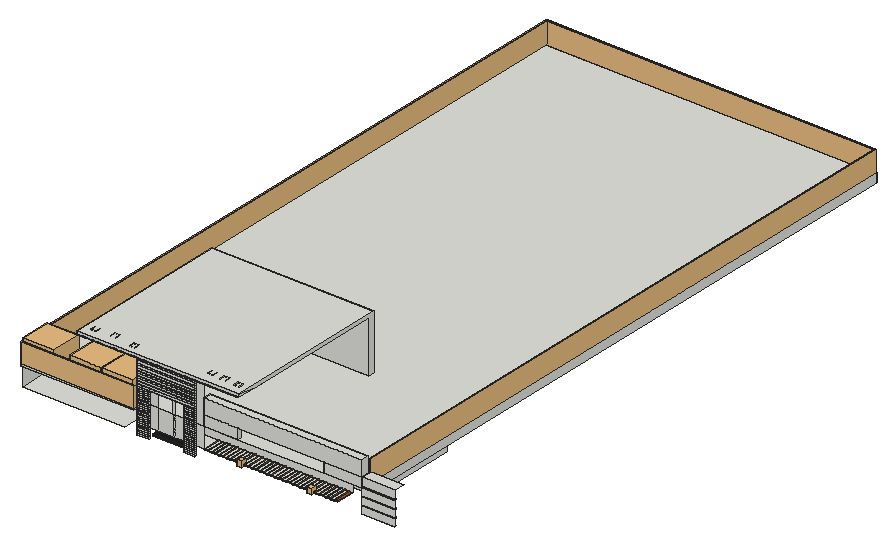
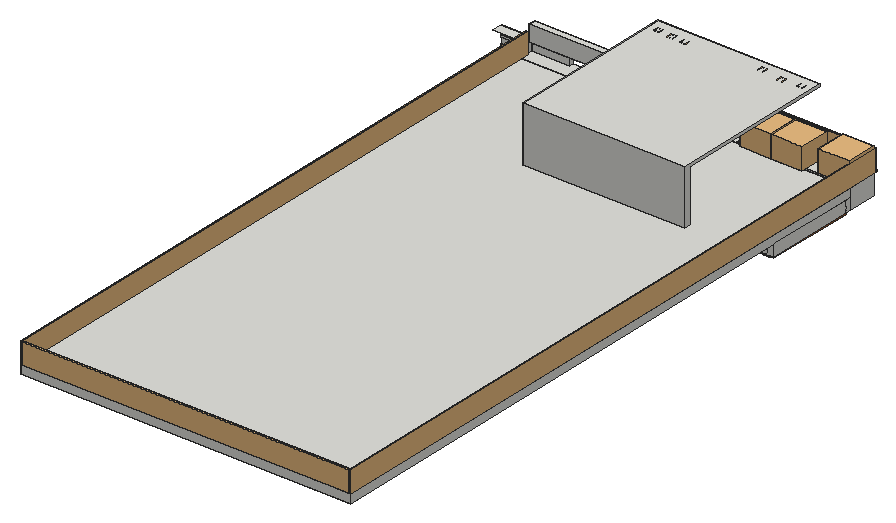
# SketchUp Ruby script. Lengths in inches.
U = 1.inch
M = Sketchup.active_model
def pt(a) = Geom::Point3d.new(a.map { |v| v * U })
def face(e, loops, mat)
  f = e.add_face(loops[0].map { |a| pt(a) })
  loops[1..].each { |l| e.add_face(l.map { |a| pt(a) }).erase! }
  f.material = f.back_material = mat if mat
  f
end
# faces: each face lists its corners as indices into pts; further lists are holes
def faces(e, pts, list, mat = nil) = list.each { |f| face(e, (f[0].is_a?(Array) ? f : [f]).map { |l| l.map { |i| pts[i] } }, mat) }
# xy, xz, yz: faces in a plane at the given z, y or x. An outline is a flat list of corners, or four numbers for a rectangle; further outlines are holes
def ring(l) = l.size == 4 ? [[l[0], l[1]], [l[2], l[1]], [l[2], l[3]], [l[0], l[3]]] : l.each_slice(2).to_a
def flat(e, list, mat, &to3) = list.each { |f| face(e, (f[0].is_a?(Array) ? f : [f]).map { |l| ring(l).map { |u, v| to3.(u, v) } }, mat) }
def xy(e, z, list, mat = nil) = flat(e, list, mat) { |x, y| [x, y, z] }
def xz(e, y, list, mat = nil) = flat(e, list, mat) { |x, z| [x, y, z] }
def yz(e, x, list, mat = nil) = flat(e, list, mat) { |y, z| [x, y, z] }
def lines(e, pts, list) = list.each { |a, b| e.add_line(pt(pts[a]), pt(pts[b])) }
# prism: a flat outline (further loops are holes) pulled along v
def prism(e, loops, v, mat = nil)
  f = face(e, loops, mat); d = Geom::Vector3d.new(v.map { |x| x * U })
  f.pushpull(f.normal.samedirection?(d) ? d.length : -d.length)
end
def box(e, o, s, mat = nil) = prism(e, [[o, [o[0] + s[0], o[1], o[2]], [o[0] + s[0], o[1] + s[1], o[2]], [o[0], o[1] + s[1], o[2]]]], [0, 0, s[2]], mat)
def at(x, y, z, deg = 0) = Geom::Transformation.translation(pt([x, y, z])) * Geom::Transformation.rotation(ORIGIN, Z_AXIS, deg.degrees)
def axes(o, x, y, z) = Geom::Transformation.new([*x, 0, *y, 0, *z, 0, *pt(o).to_a, 1])
def part(name) = M.definitions.add(name)
# library, detail: a bought-in or finely detailed component or shape, given as its bounding box
def library(name, o, s) = part(name).tap { |d| box(d.entities, o, s) }
def detail(e, o, s) = box(e.add_group.entities, o, s)
def put(e, d, t, mat = nil) = e.add_instance(d, t).tap { |i| i.material = mat if mat }
def group(e, t, mat = nil) = e.add_group.tap { |g| g.transformation = t; g.material = mat if mat }.entities
root = M.entities
M.materials.add("[Color M08]").color = [30, 30, 30]
M.materials.add("[Wood Cherry Original]").color = [152, 86, 42]
c1 = library("Untitled",[-42.57,156.8,-6.73],[9.02,9.02,10.27])
c2 = part("Group\#7")
box(c2.entities,[0,-1.25,0],[16.29,1.25,1.96])
c3 = part("Group\#6")
box(c3.entities,[0,-1.25,0],[15.54,1.25,1.96])
c4 = part("Group\#9")
box(c4.entities,[0,0,-1.4375],[4.4375,120.65,1.4375])
c5 = part("Group\#8")
box(c5.entities,[0,0,-1.0625],[4.43,24.5,1.0625])
c6 = library("Glass Railings(black Handrails)",[-57.04,-132.55,0],[169.29,2.52,28.17])
c7 = library("plant",[8.5625,309.59,291.73],[41.91,41.15,29.33])
c8 = part("Group\#5")
box(c8.entities,[0,-1.25,0],[78.66,1.25,2.55])
c9 = part("Group\#16")
box(c9.entities,[0,0,-0.25],[2.67,219.03,0.25])
xy(root,233.38,[[506,180.5,550.5625,182.5]])
xy(root,233.875,[[231.53,172.8125,279.16,180.5]])
xy(root,235.5625,[[68.72,225.73,82.03,242.29]])
xy(root,237,[[62,164.8125,199.16,205],[215,180.5,469.32,205],[62,205,208.8125,213.35],[208.8125,205,215,213.35],[66.4375,213.35,66.4375,334,497,334,497,214,208.8125,214,208.8125,213.35],
  [208.8125,213.35,215,214]])
xy(root,237,[[231.53,172.8125,279.16,180.5]],"[Color M08]")
xy(root,242.38,[[506,180.5,550.5625,182.5]])
xy(root,244.38,[[506,180.5,550.5625,182.5]])
xy(root,252.4375,[[62,205,215,213.35],[[215,205,506,205,506,1045,62,1045,62,334,497,334,497,213.35,215,213.35],[219,338,219,522,243,522,243,730,239,730,239,526,71,526,71,800,179,800,179,734,183,734,183,864,237,864,237,936,373,936,373,806,418,806,418,758,349,758,349,582,397,582,397,522,349,522,349,338],[71,868,233,1036],[71,338,215,522],[353,338,497,518],[353,586,497,754],[377,892,497,1036],[377,810,497,888],[301,940,373,1036],[71,804,179,864],[401,522,497,582],[237,940,297,1036],[422,758,497,806]],[215,213.35,497,214],[71,730,183,734],[183,730,243,734]])
xy(root,253.38,[[506,180.5,550.5625,182.5]])
xy(root,255.38,[[506,180.5,550.5625,182.5]])
xy(root,264.38,[[506,180.5,550.5625,182.5]])
xy(root,264.4375,[[62,161.3125,215,164.8125],[62,164.8125,215,205],[215,180.5,293.91,180.5,293.91,185.8125,339.47,185.8125,339.47,180.5,454.8125,180.5,454.8125,185.8125,506,185.8125,506,205,215,205],[293.91,180.5,339.47,185.8125],[454.8125,180.5,506,185.8125],
  [143.43,372.84,361.41,381.625]])
xy(root,265.8125,[[62,161.3125,215,205]])
xy(root,266.38,[[506,180.5,550.5625,182.5]])
xy(root,277.75,[[293.91,180.5,339.47,185.8125],[339.47,180.5,454.8125,190.4375],[454.8125,180.5,506,185.8125],[506,180.5,550.5625,195.0625],[293.91,185.8125,339.47,190.4375],
  [454.8125,185.8125,506,190.4375]])
xy(root,292.39,[[252.06,176.36,254.95,180.5]])
xy(root,292.78,[[231.53,166.5625,278.36,180.5]])
xy(root,298.6875,[[293.91,180.5,506,190.4375]])
xy(root,334.5625,[[146.11,153.8125,146.11,372.84,361.41,372.84,361.41,180.5,215.24,180.5,215.24,153.8125],[294.08,153.8125,293.91,166.5625,293.91,180.5,361.41,180.5,361.58,153.8125]])
xy(root,334.5625,[[215.24,153.8125,294.08,153.8125,293.91,166.5625,293.91,180.5,215.24,180.5]],"[Wood Cherry Original]")
xy(root,338.125,[[143.43,153.8125,361.41,381.625]])
xz(root,153.8125,[[143.43,334.5625,361.58,334.5625,361.41,338.125,143.43,338.125]])
xz(root,161.3125,[[62,264.4375,215,265.8125]])
xz(root,172.8125,[[231.53,233.875,279.16,237]],"[Color M08]")
xz(root,180.5,[[506,233.38,550.5625,242.38],[252.06,233.875,254.95,237],[254.95,233.875,278.36,237],[278.36,233.875,279.16,237],[215,237,215.24,264.4375],
  [215.24,237,231.53,264.4375],[231.53,237,252.06,264.4375],[252.06,237,254.95,264.4375],[254.95,237,278.36,264.4375],[278.36,237,293.91,264.4375],
  [506,244.38,550.5625,253.38],[506,255.38,550.5625,264.38],[215.24,264.4375,215.24,334.5625,293.91,334.5625,293.91,264.4375,278.36,264.4375,278.36,292.78,231.53,292.78,231.53,264.4375],[252.06,264.4375,254.95,292.39],[293.91,264.4375,339.47,277.75],
  [454.8125,264.4375,506,277.75],[506,266.38,550.5625,277.75],[293.91,277.75,506,298.6875]])
xz(root,182.5,[[506,242.38,550.5625,244.38],[506,253.38,550.5625,255.38],[506,264.38,550.5625,266.38]])
xz(root,185.8125,[[293.91,264.4375,339.47,277.75],[454.8125,264.4375,506,277.75]])
xz(root,190.4375,[[293.91,277.75,506,298.6875]])
xz(root,205,[[62,237,215,252.4375],[215,237,473.75,252.4375],[62,252.4375,215,264.4375],[215,252.4375,506,264.4375],[62,264.4375,215,265.8125]])
xz(root,213.35,[[62,237,215,252.4375]])
xz(root,214,[[215,237,497,252.4375]])
xz(root,334,[[62,237,71,252.4375],[71,237,497,252.4375]])
xz(root,372.84,[[143.43,264.4375,361.41,334.5625]])
xz(root,381.625,[[143.43,264.4375,361.41,338.125]])
yz(root,62,[[164.8125,237,205,264.4375],[205,237,213.35,252.4375],[213.35,237,334,252.4375],[161.3125,264.4375,205,265.8125]])
yz(root,143.43,[[372.84,264.4375,372.84,334.5625,153.8125,334.5625,153.8125,338.125,381.625,338.125,381.625,264.4375]])
yz(root,215,[[205,237,213.35,252.4375],[213.35,237,214,252.4375],[161.3125,264.4375,180.5,265.8125],[180.5,264.4375,205,265.8125]])
yz(root,279.16,[[172.8125,233.875,180.5,237]])
yz(root,293.91,[[180.5,264.4375,185.8125,277.75],[180.5,277.75,190.4375,298.6875]])
yz(root,339.47,[[180.5,264.4375,185.8125,277.75]])
yz(root,361.41,[[372.84,264.4375,381.625,264.4375,381.625,338.125,153.8125,338.125,180.5,334.5625,372.84,334.5625]])
yz(root,454.8125,[[180.5,264.4375,185.8125,277.75]])
yz(root,497,[[214,237,334,252.4375]])
yz(root,506,[[180.5,242.38,182.5,244.38],[180.5,253.38,182.5,255.38],[180.5,264.38,182.5,264.4375],[180.5,264.4375,182.5,266.38],[182.5,264.4375,182.5,266.38,180.5,266.38,180.5,277.75,185.8125,277.75,185.8125,264.4375],
  [185.8125,264.4375,195.0625,277.75],[180.5,277.75,190.4375,298.6875]])
p = [[361.58,153.8125,334.5625],[361.41,180.5,334.5625],[361.41,153.8125,338.125]]
faces(root,p,[[0,1,2]])
put(root,c1,axes([370.95,60.24,238.25],[0.76,0,0],[0,0.76,0],[0,0,0.76]))
put(root,c1,axes([125.42,104.8125,238.3],[0.76,0,0],[0,0.76,0],[0,0,0.76]))
put(root,c1,axes([174.55,104.8125,238.3],[0.76,0,0],[0,0.76,0],[0,0,0.76]))
put(root,c1,axes([223.22,104.8125,238.3],[0.76,0,0],[0,0.76,0],[0,0,0.76]))
put(root,c1,axes([129.81,196.9,238.3],[0.76,0,0],[0,0.76,0],[0,0,0.76]))
put(root,c1,axes([227.61,196.9,238.3],[0.76,0,0],[0,0.76,0],[0,0,0.76]))
put(root,c1,axes([178.93,196.9,238.3],[0.76,0,0],[0,0.76,0],[0,0,0.76]))
put(root,c1,axes([465.01,60.24,238.37],[0.76,0,0],[0,0.76,0],[0,0,0.76]))
put(root,c2,at(215.24,166.5625,233.46))
put(root,c3,at(278.36,166.5625,234.22))
put(root,c4,at(62,213.35,237),"[Wood Cherry Original]")
put(root,c4,at(68.72,213.35,237),"[Wood Cherry Original]")
put(root,c4,at(75.28,213.35,237),"[Wood Cherry Original]")
put(root,c4,at(82.03,213.35,237),"[Wood Cherry Original]")
put(root,c4,at(88.59,213.35,237),"[Wood Cherry Original]")
put(root,c4,at(94.34,213.35,237),"[Wood Cherry Original]")
put(root,c4,at(100.84,213.35,237),"[Wood Cherry Original]")
put(root,c4,at(106.84,213.35,237),"[Wood Cherry Original]")
put(root,c4,at(113.03,213.35,237),"[Wood Cherry Original]")
put(root,c4,at(119.53,213.35,237),"[Wood Cherry Original]")
put(root,c4,at(126.03,213.35,237),"[Wood Cherry Original]")
put(root,c4,at(133.66,213.35,237),"[Wood Cherry Original]")
put(root,c4,at(140.53,213.35,237),"[Wood Cherry Original]")
put(root,c4,at(147.97,213.35,237),"[Wood Cherry Original]")
put(root,c4,at(156.03,213.35,237),"[Wood Cherry Original]")
put(root,c4,at(164.22,213.35,237),"[Wood Cherry Original]")
put(root,c4,at(171.53,213.35,237),"[Wood Cherry Original]")
put(root,c4,at(179.84,213.35,237),"[Wood Cherry Original]")
put(root,c4,at(186.28,213.35,237),"[Wood Cherry Original]")
put(root,c4,at(193.16,213.35,237),"[Wood Cherry Original]")
put(root,c4,at(200.97,213.35,237),"[Wood Cherry Original]")
put(root,c4,at(207.59,213.35,237),"[Wood Cherry Original]")
put(root,c4,at(215.91,213.35,237),"[Wood Cherry Original]")
put(root,c4,at(224.72,213.35,237),"[Wood Cherry Original]")
put(root,c4,at(233.16,213.35,237),"[Wood Cherry Original]")
put(root,c4,at(241.78,213.35,237),"[Wood Cherry Original]")
put(root,c2,at(215.24,166.5625,235.65))
put(root,c5,at(469.32,180.5,237),"[Wood Cherry Original]")
put(root,c5,at(464.07,180.5,237),"[Wood Cherry Original]")
put(root,c5,at(458.7,180.5,237),"[Wood Cherry Original]")
put(root,c5,at(453.57,180.5,237),"[Wood Cherry Original]")
put(root,c5,at(448.51,180.5,237),"[Wood Cherry Original]")
put(root,c5,at(443.42,180.5,237),"[Wood Cherry Original]")
put(root,c5,at(438.48,180.5,237),"[Wood Cherry Original]")
put(root,c5,at(433.48,180.5,237),"[Wood Cherry Original]")
put(root,c5,at(428.54,180.5,237),"[Wood Cherry Original]")
put(root,c5,at(423.6,180.5,237),"[Wood Cherry Original]")
put(root,c5,at(418.6,180.5,237),"[Wood Cherry Original]")
put(root,c5,at(413.79,180.5,237),"[Wood Cherry Original]")
put(root,c5,at(408.92,180.5,237),"[Wood Cherry Original]")
put(root,c5,at(404.04,180.5,237),"[Wood Cherry Original]")
put(root,c5,at(398.98,180.5,237),"[Wood Cherry Original]")
put(root,c5,at(393.92,180.5,237),"[Wood Cherry Original]")
put(root,c5,at(388.85,180.5,237),"[Wood Cherry Original]")
put(root,c5,at(383.85,180.5,237),"[Wood Cherry Original]")
put(root,c5,at(378.92,180.5,237),"[Wood Cherry Original]")
put(root,c5,at(374.23,180.5,237),"[Wood Cherry Original]")
put(root,c5,at(369.23,180.5,237),"[Wood Cherry Original]")
put(root,c5,at(364.04,180.5,237),"[Wood Cherry Original]")
put(root,c5,at(358.73,180.5,237),"[Wood Cherry Original]")
put(root,c5,at(353.48,180.5,237),"[Wood Cherry Original]")
put(root,c5,at(348.1,180.5,237),"[Wood Cherry Original]")
put(root,c5,at(343.23,180.5,237),"[Wood Cherry Original]")
put(root,c5,at(338.29,180.5,237),"[Wood Cherry Original]")
put(root,c5,at(333.48,180.5,237),"[Wood Cherry Original]")
put(root,c5,at(328.67,180.5,237),"[Wood Cherry Original]")
put(root,c5,at(323.92,180.5,237),"[Wood Cherry Original]")
put(root,c5,at(318.92,180.5,237),"[Wood Cherry Original]")
put(root,c5,at(314.17,180.5,237),"[Wood Cherry Original]")
put(root,c5,at(309.23,180.5,237),"[Wood Cherry Original]")
put(root,c5,at(304.23,180.5,237),"[Wood Cherry Original]")
put(root,c5,at(299.3,180.5,237),"[Wood Cherry Original]")
put(root,c5,at(294.3,180.5,237),"[Wood Cherry Original]")
put(root,c3,at(278.36,166.5625,236.41))
put(root,c2,at(215.24,166.5625,237.84))
put(root,c3,at(278.36,166.5625,238.78))
put(root,c2,at(215.24,166.5625,240.02))
put(root,c3,at(278.36,166.5625,241.03))
put(root,c2,at(215.24,166.5625,242.27))
put(root,c3,at(278.36,166.5625,243.35))
put(root,c2,at(215.24,166.5625,244.46))
put(root,c3,at(278.36,166.5625,245.66))
put(root,c2,at(215.24,166.5625,246.65))
put(root,c3,at(278.36,166.5625,247.97))
put(root,c2,at(215.24,166.5625,249.02))
put(root,c3,at(278.36,166.5625,250.35))
put(root,c2,at(215.24,166.5625,251.34))
g1 = group(root,at(62,1045,252.4375))
box(g1,[0,-840,0],[444,840,12])
put(root,c3,at(278.36,166.5625,252.66))
put(root,c2,at(215.24,166.5625,253.65))
put(root,c3,at(278.36,166.5625,254.97))
put(root,c2,at(215.24,166.5625,255.84))
put(root,c3,at(278.36,166.5625,257.28))
put(root,c2,at(215.24,166.5625,258.02))
put(root,c3,at(278.36,166.5625,259.59))
put(root,c2,at(215.24,166.5625,260.27))
put(root,c3,at(278.36,166.5625,261.84))
put(root,c2,at(215.24,166.5625,262.46))
put(root,c3,at(278.36,166.5625,264.09))
put(root,c6,axes([636.03,758.68,264.43],[0,-5.01924,0],[1,0,0],[0,0,1]))
put(root,c6,axes([113.33,294.47,264.4375],[0.9,0,0],[0,1,0],[0,0,1]))
put(root,c6,axes([194.5,748.36,264.4375],[0,-5.20008,0],[1,0,0],[0,0,1]))
put(root,c6,axes([212.03,1175.41,264.4375],[2.60007,0,0],[0,1,0],[0,0,1]))
put(root,c2,at(215.24,166.5625,264.65))
put(root,c7,at(156.58,-140.6,-26.46))
put(root,c7,at(113.9,-140.6,-26.46))
put(root,c3,at(278.36,166.5625,266.46))
put(root,c2,at(215.24,166.5625,266.9))
put(root,c7,at(54.04,-145.06,-24.57))
put(root,c3,at(278.36,166.5625,268.77))
put(root,c2,at(215.24,166.5625,269.09))
put(root,c3,at(278.36,166.5625,271.15))
put(root,c2,at(215.24,166.5625,271.27))
put(root,c3,at(278.36,166.5625,273.4))
put(root,c2,at(215.24,166.5625,273.46))
put(root,c2,at(215.24,166.5625,275.71))
put(root,c3,at(278.36,166.5625,275.77))
put(root,c2,at(215.24,166.5625,278.02))
put(root,c3,at(278.36,166.5625,278.02))
put(root,c2,at(215.24,166.5625,280.27))
put(root,c3,at(278.36,166.5625,280.46))
put(root,c2,at(215.24,166.5625,282.59))
put(root,c3,at(278.36,166.5625,282.84))
put(root,c2,at(215.24,166.5625,284.9))
put(root,c3,at(278.36,166.5625,285.21))
put(root,c2,at(215.24,166.5625,287.34))
put(root,c3,at(278.36,166.5625,287.52))
put(root,c2,at(215.24,166.5625,289.77))
put(root,c3,at(278.36,166.5625,289.77))
put(root,c8,at(215.24,166.5625,292.39))
put(root,c8,at(215.24,166.5625,295.51))
put(root,c8,at(215.24,166.5625,298.58))
put(root,c8,at(215.24,166.5625,301.83))
put(root,c8,at(215.24,166.5625,304.83))
put(root,c8,at(215.24,166.5625,307.83))
put(root,c8,at(215.24,166.5625,310.95))
put(root,c8,at(215.24,166.5625,314.14))
put(root,c8,at(215.24,166.5625,317.14))
put(root,c8,at(215.24,166.5625,320.14))
put(root,c8,at(215.24,166.5625,323.01))
put(root,c8,at(215.24,166.5625,325.95))
put(root,c8,at(215.24,166.5625,328.95))
put(root,c1,axes([185.36,46.71,335.43],[0.76,0,0],[0,0.76,0],[0,0,0.76]))
put(root,c1,axes([209.96,49.1875,335.43],[0.76,0,0],[0,0.76,0],[0,0,0.76]))
put(root,c1,axes([239.12,44.52,335.43],[0.76,0,0],[0,0.76,0],[0,0,0.76]))
put(root,c1,axes([339.625,50.17,335.43],[0.76,0,0],[0,0.76,0],[0,0,0.76]))
put(root,c1,axes([357.58,49.1,335.43],[0.76,0,0],[0,0.76,0],[0,0,0.76]))
put(root,c1,axes([377.28,47.5,335.43],[0.76,0,0],[0,0.76,0],[0,0,0.76]))
put(root,c8,at(215.24,166.5625,332.01))
put(root,c9,at(143.43,153.8125,334.5625),"[Wood Cherry Original]")
put(root,c9,at(146.31,153.8125,334.5625),"[Wood Cherry Original]")
put(root,c9,at(149.24,153.8125,334.5625),"[Wood Cherry Original]")
put(root,c9,at(152.24,153.8125,334.5625),"[Wood Cherry Original]")
put(root,c9,at(155.18,153.8125,334.5625),"[Wood Cherry Original]")
put(root,c9,at(158.12,153.8125,334.5625),"[Wood Cherry Original]")
put(root,c9,at(161.06,153.8125,334.5625),"[Wood Cherry Original]")
put(root,c9,at(163.93,153.8125,334.5625),"[Wood Cherry Original]")
put(root,c9,at(166.81,153.8125,334.5625),"[Wood Cherry Original]")
put(root,c9,at(169.62,153.8125,334.5625),"[Wood Cherry Original]")
put(root,c9,at(172.49,153.8125,334.5625),"[Wood Cherry Original]")
put(root,c9,at(175.37,153.8125,334.5625),"[Wood Cherry Original]")
put(root,c9,at(178.18,153.8125,334.5625),"[Wood Cherry Original]")
put(root,c9,at(180.99,153.8125,334.5625),"[Wood Cherry Original]")
put(root,c9,at(183.93,153.8125,334.5625),"[Wood Cherry Original]")
put(root,c9,at(186.81,153.8125,334.5625),"[Wood Cherry Original]")
put(root,c9,at(189.62,153.8125,334.5625),"[Wood Cherry Original]")
put(root,c9,at(192.49,153.8125,334.5625),"[Wood Cherry Original]")
put(root,c9,at(195.24,153.8125,334.5625),"[Wood Cherry Original]")
put(root,c9,at(198.12,153.8125,334.5625),"[Wood Cherry Original]")
put(root,c9,at(200.93,153.8125,334.5625),"[Wood Cherry Original]")
put(root,c9,at(203.74,153.8125,334.5625),"[Wood Cherry Original]")
put(root,c9,at(206.62,153.8125,334.5625),"[Wood Cherry Original]")
put(root,c9,at(209.43,153.8125,334.5625),"[Wood Cherry Original]")
put(root,c9,at(212.24,153.8125,334.5625),"[Wood Cherry Original]")
put(root,c9,at(214.99,153.8125,334.5625),"[Wood Cherry Original]")
put(root,c9,at(217.81,153.8125,334.5625),"[Wood Cherry Original]")
put(root,c9,at(220.62,153.8125,334.5625),"[Wood Cherry Original]")
put(root,c9,at(223.43,153.8125,334.5625),"[Wood Cherry Original]")
put(root,c9,at(226.24,153.8125,334.5625),"[Wood Cherry Original]")
put(root,c9,at(229.06,153.8125,334.5625),"[Wood Cherry Original]")
put(root,c9,at(231.87,153.8125,334.5625),"[Wood Cherry Original]")
put(root,c9,at(234.74,153.8125,334.5625),"[Wood Cherry Original]")
put(root,c9,at(237.56,153.8125,334.5625),"[Wood Cherry Original]")
put(root,c9,at(240.43,153.8125,334.5625),"[Wood Cherry Original]")
put(root,c9,at(243.31,153.8125,334.5625),"[Wood Cherry Original]")
put(root,c9,at(246.12,153.8125,334.5625),"[Wood Cherry Original]")
put(root,c9,at(248.93,153.8125,334.5625),"[Wood Cherry Original]")
put(root,c9,at(251.81,153.8125,334.5625),"[Wood Cherry Original]")
put(root,c9,at(254.57,153.8125,334.5625),"[Wood Cherry Original]")
put(root,c9,at(257.51,153.8125,334.5625),"[Wood Cherry Original]")
put(root,c9,at(260.45,153.8125,334.5625),"[Wood Cherry Original]")
put(root,c9,at(263.26,153.8125,334.5625),"[Wood Cherry Original]")
put(root,c9,at(266.2,153.8125,334.5625),"[Wood Cherry Original]")
put(root,c9,at(269.2,153.8125,334.5625),"[Wood Cherry Original]")
put(root,c9,at(272.26,153.8125,334.5625),"[Wood Cherry Original]")
put(root,c9,at(275.26,153.8125,334.5625),"[Wood Cherry Original]")
put(root,c9,at(278.26,153.8125,334.5625),"[Wood Cherry Original]")
put(root,c9,at(281.57,153.8125,334.5625),"[Wood Cherry Original]")
put(root,c9,at(284.57,153.8125,334.5625),"[Wood Cherry Original]")
put(root,c9,at(287.7,153.8125,334.5625),"[Wood Cherry Original]")
put(root,c9,at(290.7,153.8125,334.5625),"[Wood Cherry Original]")
put(root,c9,at(293.91,153.8125,334.5625),"[Wood Cherry Original]")
put(root,c9,at(297.03,153.8125,334.5625),"[Wood Cherry Original]")
put(root,c9,at(300.03,153.8125,334.5625),"[Wood Cherry Original]")
put(root,c9,at(302.84,153.8125,334.5625),"[Wood Cherry Original]")
put(root,c9,at(305.72,153.8125,334.5625),"[Wood Cherry Original]")
put(root,c9,at(308.59,153.8125,334.5625),"[Wood Cherry Original]")
put(root,c9,at(311.53,153.8125,334.5625),"[Wood Cherry Original]")
put(root,c9,at(314.47,153.8125,334.5625),"[Wood Cherry Original]")
put(root,c9,at(317.28,153.8125,334.5625),"[Wood Cherry Original]")
put(root,c9,at(320.22,153.8125,334.5625),"[Wood Cherry Original]")
put(root,c9,at(323.22,153.8125,334.5625),"[Wood Cherry Original]")
put(root,c9,at(326.03,153.8125,334.5625),"[Wood Cherry Original]")
put(root,c9,at(328.91,153.8125,334.5625),"[Wood Cherry Original]")
put(root,c9,at(331.78,153.8125,334.5625),"[Wood Cherry Original]")
put(root,c9,at(334.66,153.8125,334.5625),"[Wood Cherry Original]")
put(root,c9,at(337.59,153.8125,334.5625),"[Wood Cherry Original]")
put(root,c9,at(340.47,153.8125,334.5625),"[Wood Cherry Original]")
put(root,c9,at(343.34,153.8125,334.5625),"[Wood Cherry Original]")
put(root,c9,at(346.22,153.8125,334.5625),"[Wood Cherry Original]")
put(root,c9,at(349.09,153.8125,334.5625),"[Wood Cherry Original]")
put(root,c9,at(352.03,153.8125,334.5625),"[Wood Cherry Original]")
put(root,c9,at(354.97,153.8125,334.5625),"[Wood Cherry Original]")
put(root,c9,at(357.91,153.8125,334.5625),"[Wood Cherry Original]")
